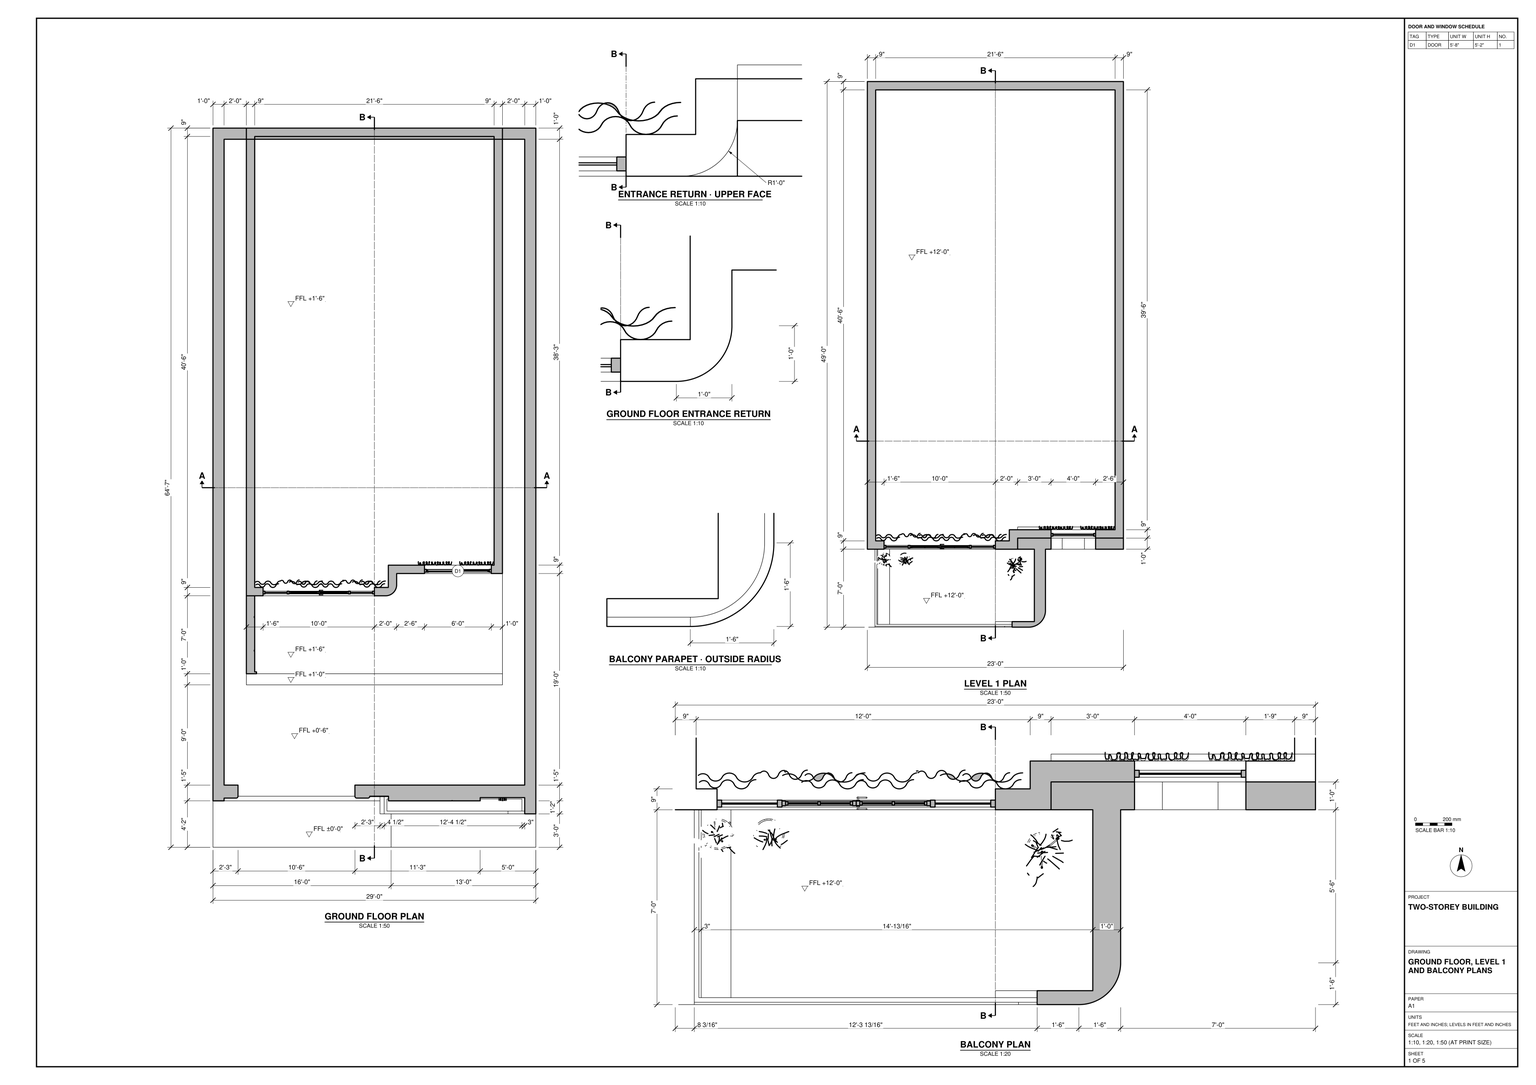
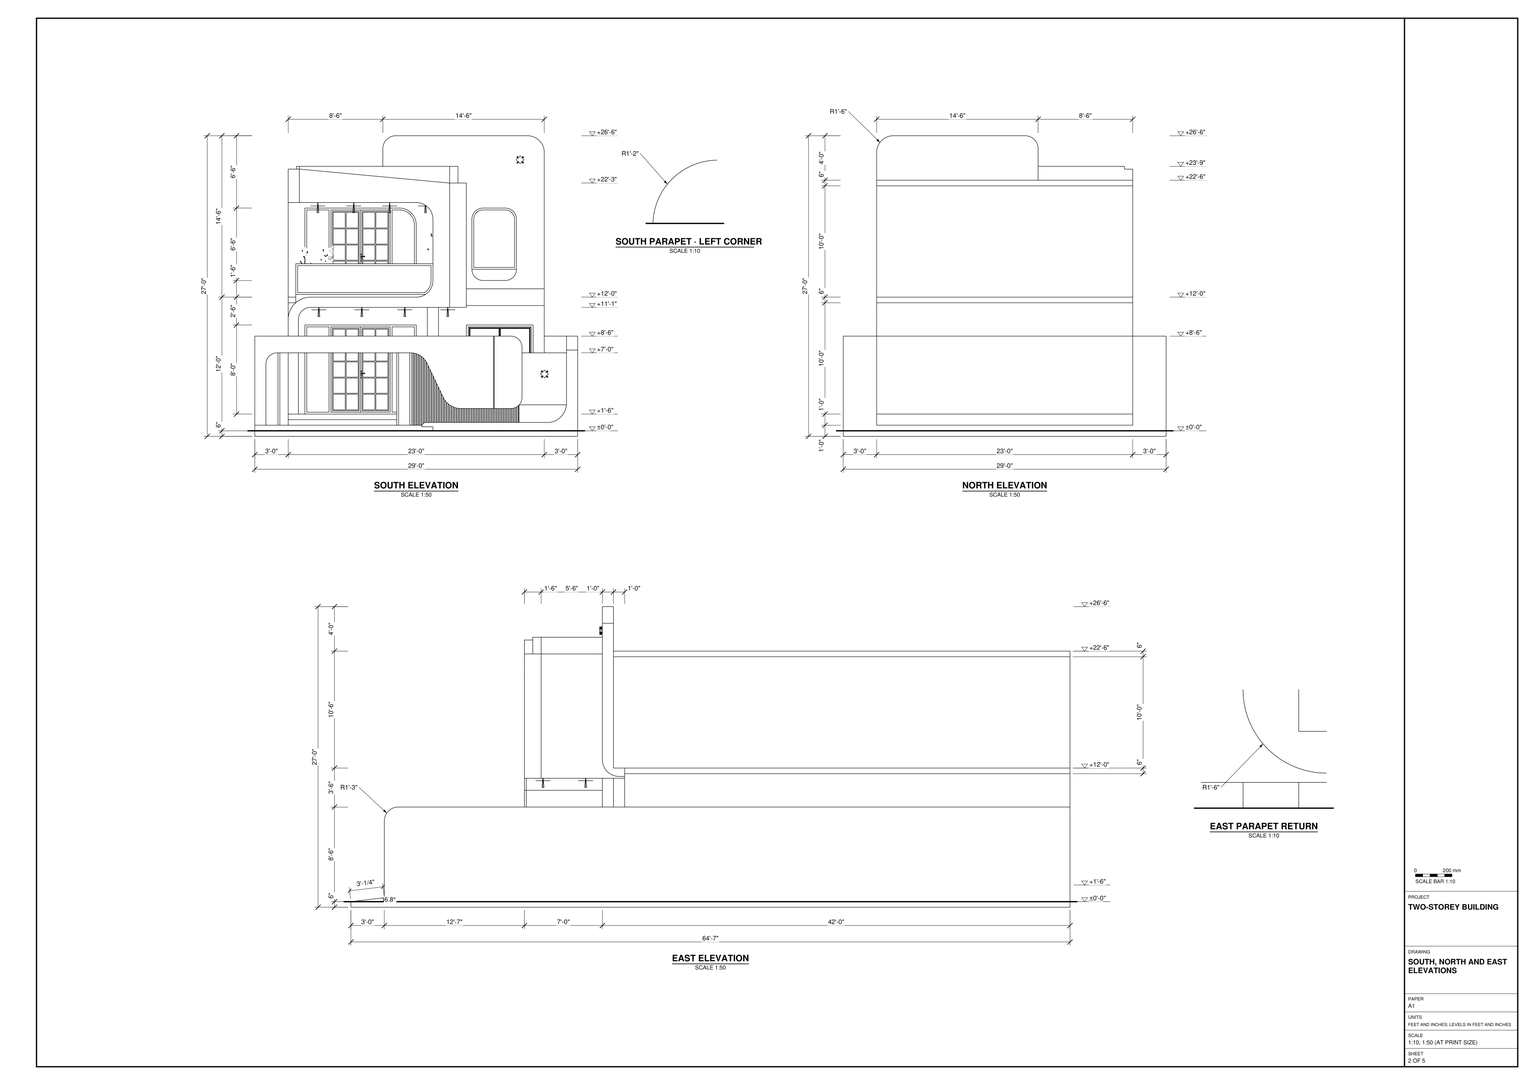
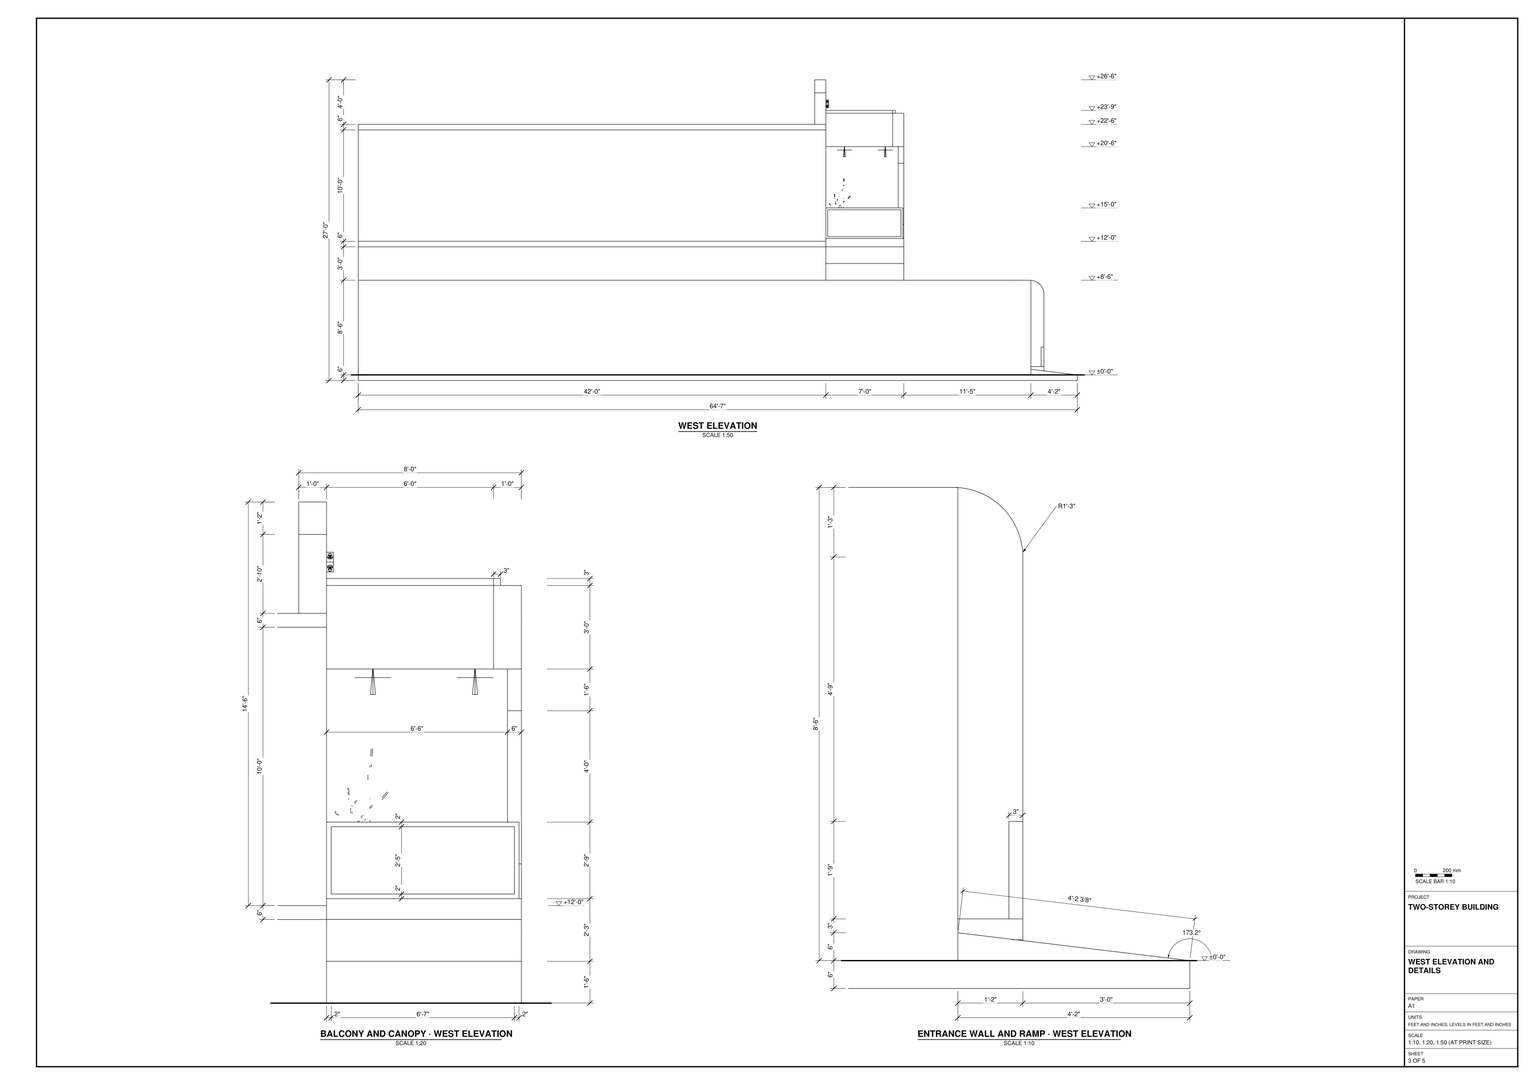
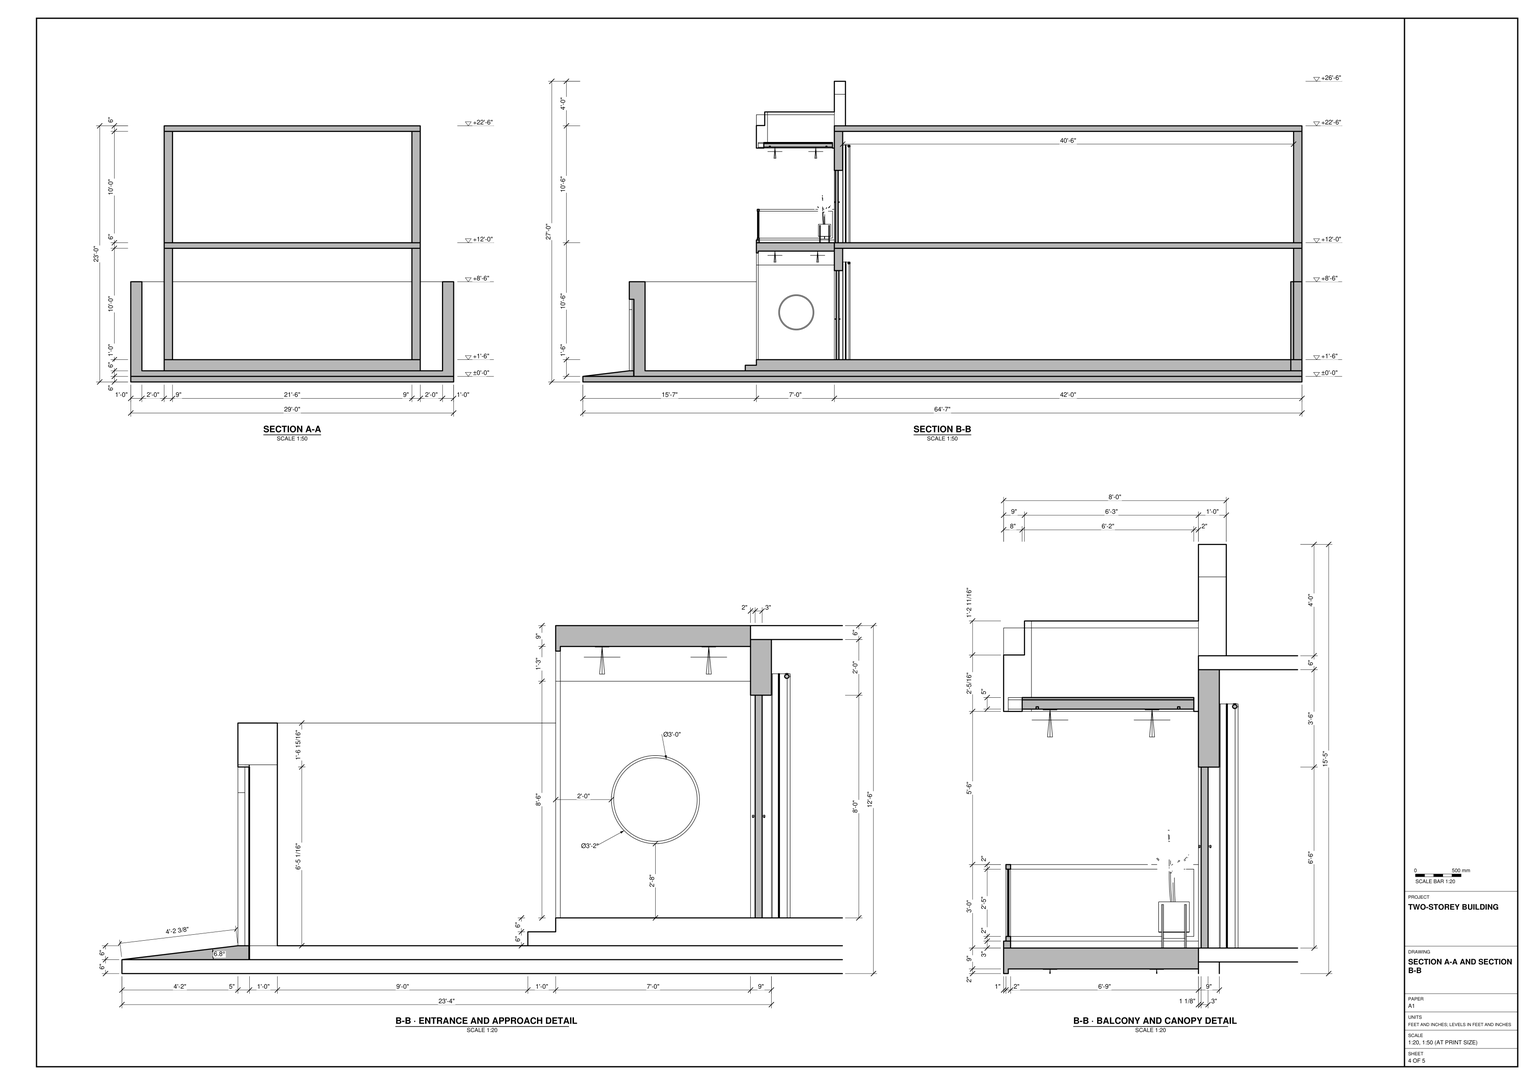
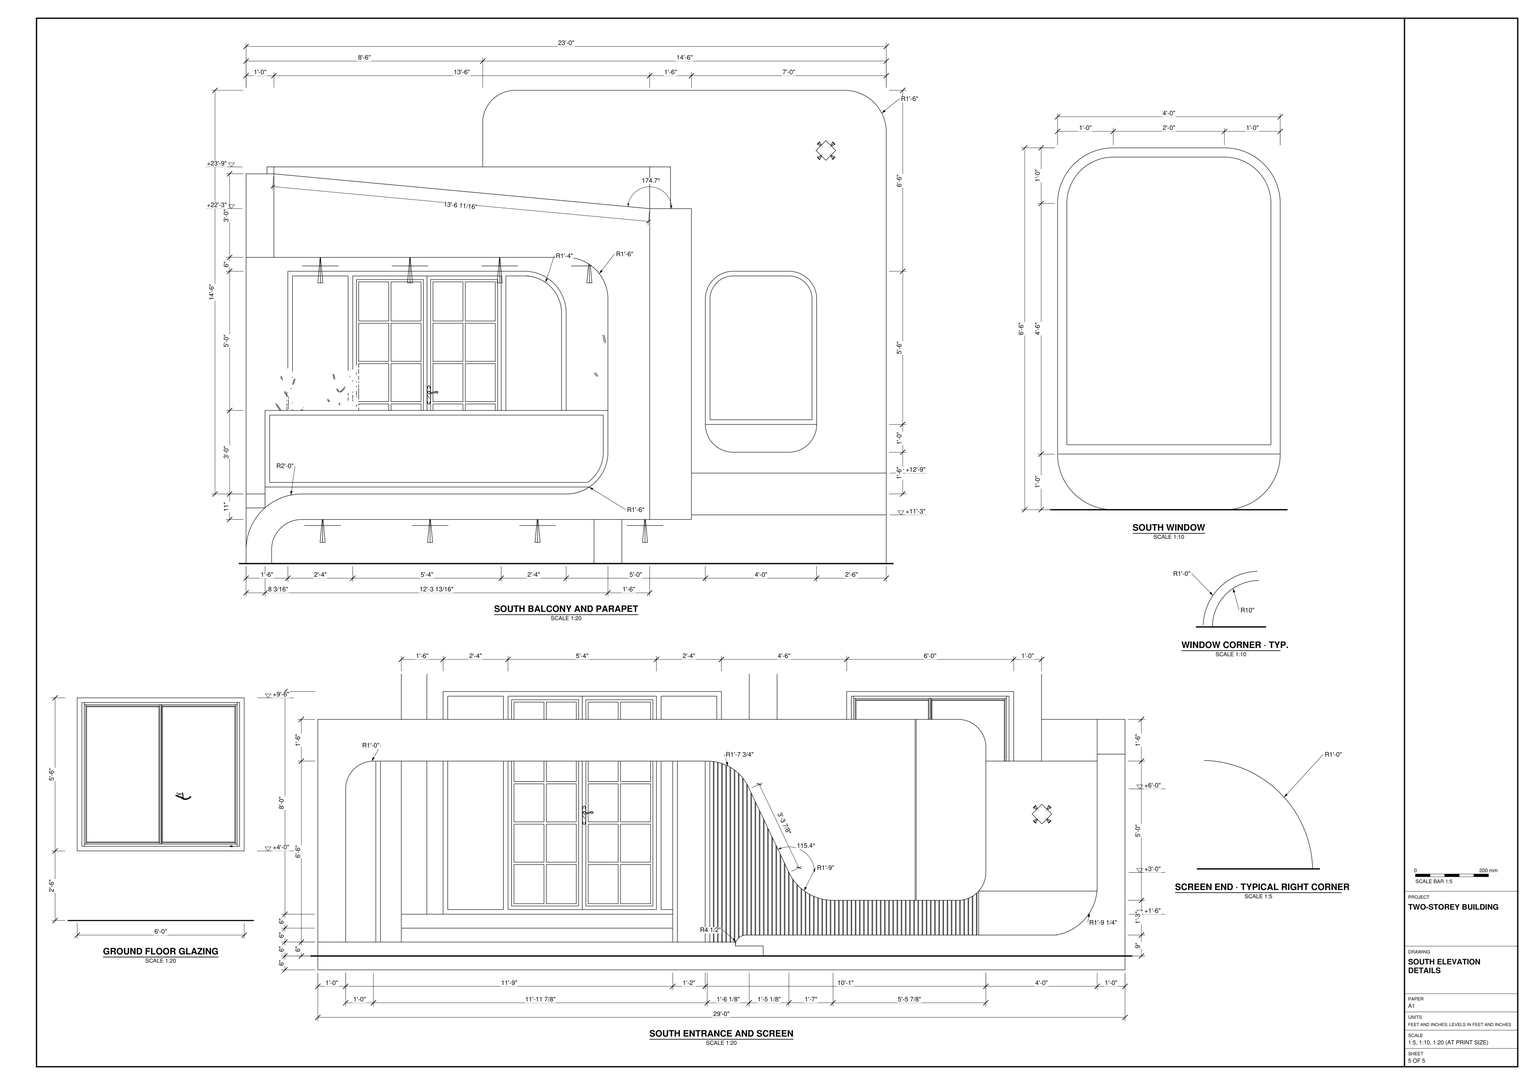
Build the two-storey building in SketchUp from task_files/diagram_01.pdf. Work in feet and inches. Set out the model 29'-0" wide by 64'-7" deep, with an overall height of 27'-0". Use ±0'-0" as the ground datum and +12'-0" for the upper floor. Distinguish the ground datum from the raised entrance floor at +1'-6".

Centre the narrower building shell between the long side boundary walls, leaving the entrance court to the south. Model the walls at their drawn thicknesses, the floor and flat roof slabs, and the stepped front wall line on each storey. Follow the approach from the ramp through the screened court entrance and up the steps to the recessed ground-floor glazing. Fit the door and window units into their openings. Above the entrance, model the projecting balcony, its rounded parapet return and the canopy. Use the south elevation to place the canopy in front of the taller parapet and the separate rounded opening beside the balcony.

Keep walls, slabs and roof in separate groups or components, group each furniture or joinery piece separately where shown, and use components for repeated parts. Decor and loose items, including balcony plants and lights, may be any suitable library components. Save one SketchUp model as output_files/two_storey_building_with_a_front_court_and_balcony.skp.

# SketchUp Ruby script. Lengths in inches.
U = 1.inch
M = Sketchup.active_model
def pt(a) = Geom::Point3d.new(a.map { |v| v * U })
def face(e, loops, mat)
  f = e.add_face(loops[0].map { |a| pt(a) })
  loops[1..].each { |l| e.add_face(l.map { |a| pt(a) }).erase! }
  f.material = f.back_material = mat if mat
  f
end
# faces: each face lists its corners as indices into pts; further lists are holes
def faces(e, pts, list, mat = nil) = list.each { |f| face(e, (f[0].is_a?(Array) ? f : [f]).map { |l| l.map { |i| pts[i] } }, mat) }
# xy, xz, yz: faces in a plane at the given z, y or x. An outline is a flat list of corners, or four numbers for a rectangle; further outlines are holes
def ring(l) = l.size == 4 ? [[l[0], l[1]], [l[2], l[1]], [l[2], l[3]], [l[0], l[3]]] : l.each_slice(2).to_a
def flat(e, list, mat, &to3) = list.each { |f| face(e, (f[0].is_a?(Array) ? f : [f]).map { |l| ring(l).map { |u, v| to3.(u, v) } }, mat) }
def xy(e, z, list, mat = nil) = flat(e, list, mat) { |x, y| [x, y, z] }
def xz(e, y, list, mat = nil) = flat(e, list, mat) { |x, z| [x, y, z] }
def yz(e, x, list, mat = nil) = flat(e, list, mat) { |y, z| [x, y, z] }
def lines(e, pts, list) = list.each { |a, b| e.add_line(pt(pts[a]), pt(pts[b])) }
# prism: a flat outline (further loops are holes) pulled along v
def prism(e, loops, v, mat = nil)
  f = face(e, loops, mat); d = Geom::Vector3d.new(v.map { |x| x * U })
  f.pushpull(f.normal.samedirection?(d) ? d.length : -d.length)
end
def box(e, o, s, mat = nil) = prism(e, [[o, [o[0] + s[0], o[1], o[2]], [o[0] + s[0], o[1] + s[1], o[2]], [o[0], o[1] + s[1], o[2]]]], [0, 0, s[2]], mat)
def at(x, y, z, deg = 0) = Geom::Transformation.translation(pt([x, y, z])) * Geom::Transformation.rotation(ORIGIN, Z_AXIS, deg.degrees)
def axes(o, x, y, z) = Geom::Transformation.new([*x, 0, *y, 0, *z, 0, *pt(o).to_a, 1])
def part(name) = M.definitions.add(name)
# library, detail: a bought-in or finely detailed component or shape, given as its bounding box
def library(name, o, s) = part(name).tap { |d| box(d.entities, o, s) }
def detail(e, o, s) = box(e.add_group.entities, o, s)
def put(e, d, t, mat = nil) = e.add_instance(d, t).tap { |i| i.material = mat if mat }
def group(e, t, mat = nil) = e.add_group.tap { |g| g.transformation = t; g.material = mat if mat }.entities
root = M.entities
M.materials.add("1421 AP 8232 ELEGANT GREY").color = [96, 96, 96]
M.materials.add("BANANA_BIG_STVOL_1").color = [93, 83, 53]
M.materials.add("POT_TEXTURE_1").color = [172, 172, 172]
M.materials.add("POT_TEXTURE_2").color = [160, 154, 144]
M.materials.add("soil1").color = [68, 55, 47]
M.materials.add("white_concrete_pot1").color = [212, 211, 204]
M.materials.add("wood_1").color = [140, 119, 94]
c1 = library("Mixed flower bed",[0,-29.95,0],[46.06,29.95,37.97])
c2 = library("Group\#85",[-312.76,2118.02,370.79],[80.37,61.43,57.53])
c3 = library("Group\#88",[-161.07,2117.49,373.61],[81.25,53.73,39.48])
c4 = library("Group\#89",[-202.35,1900.5,372.29],[58.53,80.11,50.06])
c5 = library("Group\#92",[-148.5,2084.1,354.63],[73.89,71.73,39.48])
c6 = library("Group\#94",[-392.38,2142.99,345.23],[79.77,60.6,39.05])
c7 = library("Group\#95",[-433.57,2042.61,369.7],[71.79,72.8,37.85])
c8 = library("Group\#96",[-374.28,1979.7,369.99],[51.81,82.66,37.9])
c9 = library("Group\#97",[-432.01,1984.38,372.6875],[64.1,75.95,39.0625])
c10 = library("Group\#98",[-389.63,2051.04,359.41],[56.81,81.38,37.86])
c11 = library("Group\#101",[-435.875,2067.96,347.82],[58.32,80.53,38.29])
c12 = library("Group\#102",[-362.86,1963.26,351.01],[55.56,80.44,37.9])
c13 = library("Group\#104",[-330.83,2117.69,370.2],[61.83,80.2,35.55])
c14 = library("Group\#105",[-200.52,1998.86,370.22],[77.15,68.38,35.39])
c15 = library("Group\#106",[-146.29,2044.53,349.125],[81,53.32,37.9])
c16 = library("Group\#109",[-340.96,1970.4,361.28],[81.22,51.59,61.62])
c17 = library("Group\#110",[-310.7,1952.62,354.63],[79.53,58.52,39.48])
c18 = library("Group\#111",[-143.56,2061.14,371.42],[79.79,63.19,51.3])
c19 = library("Group\#113",[-145.08,2015.32,369.99],[82.29,54.05,37.9])
c20 = library("Group\#115",[-272.7,1884.51,369.99],[80.39,55.87,37.9])
c21 = library("Group\#117",[-480.58,1843.32,11.96],[467.85,466.24,378.92])
c22 = library("Group\#120",[-363.89,1895.22,354.63],[76.92,66.54,39.48])
c23 = library("Group\#121",[-390.04,2074.71,363.78],[77.3,84.83,61.55])
c24 = library("Group\#122",[-419.21,1941.11,355.02],[73.1,71.21,39.06])
c25 = library("Group\#125",[-229.79,1894.04,351.01],[79.82,63.55,37.9])
c26 = library("Group\#127",[-397.18,1916.74,372.44],[70.02,74.57,49.25])
c27 = library("Group\#129",[-315.77,2202.04,371],[80.74,54.44,37.85])
c28 = library("Group\#131",[-372.4375,2154.5,374],[76.125,67.08,39.0625])
c29 = library("Group\#132",[-275.5,2156.34,352.11],[71.39,73.27,44.69])
c30 = library("Group\#133",[-183.79,2161.45,371.25],[72.43,70.21,54.35])
c31 = library("Group\#134",[-236.3,2186.8,344.47],[79.26,62.91,39.06])
c32 = library("Group\#135",[-366.3125,2177.8,359.41],[79.9,61.23,37.86])
c33 = library("Group\#136",[-234.26,2180.97,367.05],[50.63,74.65,43.95])
c34 = library("Group\#137",[-431.9,1883.46,368.72],[373.65,376.39,18.61])
c35 = library("Group\#138",[-904.81,1865.01,156.3],[624.43,217.34,1227.7])
c36 = library("Group\#139",[-312.51,1611.52,263.78],[120.52,408.52,1275.1])
c37 = library("Group\#140",[-571.16,1736.08,232.33],[294.08,306.57,1438.75])
c38 = library("Group\#141",[-208.23,2037.18,75.37],[621.09,225.61,1251.82])
c39 = library("Group\#142",[-273.21,1593.22,47.51],[374.54,419.07,1416.6])
c40 = library("Group\#143",[-527.15,2088.47,150.96],[267.01,328.12,1599.25])
c41 = library("Group\#144",[-675.58,1862.05,152.55],[378.81,196.01,1743.84])
c42 = library("Group\#145",[-257.06,2048.08,160.05],[394.6,177.93,1743.83])
c43 = library("Group\#146",[-344.84,1500.61,160.55],[176.35,551.19,1921.45])
c44 = library("Group\#147",[-231.77,1913.24,119.96],[448.93,143.84,1582.05])
c45 = library("Group\#148",[-616.67,2098.6,178.29],[331.19,111.16,1177.92])
c46 = library("Group\#149",[-236.03,2064.57,238.29],[378.97,266.89,1422.96])
c47 = library("Group\#150",[-792.12,2067.32,152.13],[549.56,259.52,1931.8])
c48 = library("Group\#151",[-281.17,2118.67,243.77],[133.23,408.71,1313.3])
c49 = library("Group\#152",[-468.76,669.89,380.1875],[424.36,427.47,41.99])
c50 = library("Group\#153",[-516.34,626.77,-4.5625],[517.73,515.95,418.98])
c51 = library("Group\#154",[-445.29,890.31,329.28],[284.3,304.08,2023.29])
c52 = library("Group\#155",[-277.97,488.68,287.26],[362.84,405.94,1768.54])
c53 = library("Group\#156",[-1038.76,656.55,345.34],[733.18,460.51,2065.7])
c54 = library("Group\#157",[-733.48,439.625,202.64],[456.28,533.12,1536.78])
c55 = library("Group\#158",[-249.24,914.85,310.18],[345.55,647.95,1307.93])
c56 = library("Group\#159",[-662.41,217.3,320.04],[397.32,658.3,1732.06])
c57 = library("Group\#160",[-455.56,899.32,410.78],[341.21,610.33,1581.5])
c58 = library("Group\#161",[-299.2,181.55,262.58],[360.65,735.71,1258.34])
c59 = library("Group\#162",[-258.04,-282.68,604.05],[115.53,137.01,52.63])
c60 = library("Group\#163",[-447.02,-464.95,536.35],[343.73,346.24,39.39])
c61 = library("Group\#164",[-394.9,-448.99,911.74],[90.19,96.88,85.93])
c62 = library("Group\#165",[-246.45,-349.05,558.47],[136.91,100.49,66.1])
c63 = library("Group\#166",[-249.18,-250.59,980.93],[152.21,116.16,134.05])
c64 = library("Group\#167",[-438.92,-265.61,702.3],[171.52,146.16,133.5])
c65 = library("Group\#168",[-264.68,-415.73,1484.11],[304.64,209.69,227.41])
c66 = library("Group\#169",[-545.09,-386.51,922.3125],[300.25,219.65,227.33])
c67 = library("Group\#170",[-304.79,-269.16,622.65],[82.06,111.89,102.57])
c68 = library("Group\#171",[-292.14,-288.9,1281.79],[169.55,204.34,203.36])
c69 = library("Group\#172",[-244.55,-305.59,1009.46],[103.13,76.81,77.34])
c70 = library("Group\#173",[-341.93,-403.49,744.8125],[64.83,96.32,132.15])
c71 = library("Group\#174",[-424,-312.27,817.53],[158.81,108.06,136.45])
c72 = library("Group\#175",[-357.04,-394.18,1447.05],[213.62,306.36,356.95])
c73 = library("Group\#176",[-568.91,-444.37,1285.4],[307.6,179.39,277.93])
c74 = library("Group\#177",[-388.93,-514.39,838.93],[89.79,77.73,82.08])
c75 = library("Group\#178",[-409.02,-515.05,915.53],[69.62,77.27,65.47])
c76 = library("Group\#179",[-295.03,-516.52,742.34],[68.71,141.75,78.67])
c77 = library("Group\#180",[-498.98,-524.4,908.45],[120.83,107.95,112.98])
c78 = library("Group\#181",[-278.4,-571.99,1530.91],[311.57,345.77,423.62])
c79 = library("Group\#182",[-548.25,-262.82,1459.54],[373.26,352.35,568])
c80 = library("Group\#183",[-321.08,-139.66,1308.49],[285.55,393.29,221.53])
c81 = library("Group\#184",[-387.74,-136.11,1470.07],[230,321.58,230.27])
c82 = library("Group\#185",[-293.78,-482.77,597.9],[158.75,112.78,159.87])
c83 = library("Group\#186",[-422.77,-235.4,843.61],[178.54,197.77,233.54])
c84 = library("Group\#187",[-292.81,-667.38,1418.14],[215.17,356.07,188.87])
c85 = library("Group\#188",[-385.21,-446.52,494.02],[160.93,321.12,1142.36])
c86 = library("Group\#189",[-492.14,-508.4,-4.15],[433.72,431.71,567.03])
c87 = library("Group\#190",[-429.18,-1441.17,362.05],[345.84,348.28,45.35])
c88 = library("Group\#191",[-487.23,-1483.58,-4.71],[450.86,446.99,418.38])
c89 = library("Group\#192",[-513.94,-1201.2,195.17],[480.66,557.42,1160.08])
c90 = library("Group\#193",[-545.36,-1775.03,287.125],[412.21,432,920.68])
c91 = library("Group\#194",[-208.03,-1336.63,286.21],[381.72,484.79,1145.39])
c92 = library("Group\#195",[-163.65,-1622.09,292.29],[406.18,374.8,780.12])
c93 = library("Group\#196",[-245.33,-1174.2,301.22],[356.02,306.31,608.34])
c94 = library("Group\#197",[-640.625,-1318.37,287.11],[396.64,314.81,689.96])
c95 = library("Group\#198",[-750.24,-1478.51,301.56],[423.84,451.05,998.69])
c96 = library("Group\#199",[-426.76,-1753.59,287.48],[479.67,412.35,1049.19])
c97 = library("Group\#200",[-619.83,-1636.3,288.9],[316.15,456.61,1171.28])
c98 = library("Group\#201",[-738.91,-1210.08,301],[426.4,388.88,1000.79])
c99 = library("Group\#202",[-172.82,-1329.68,294.68],[502.85,397.72,955.79])
c100 = library("Group\#203",[-208.33,-1511.76,297.04],[508.2,421.96,1258.76])
c101 = library("Group\#204",[-384.8,-1640.99,300.61],[422.68,348.03,1297.96])
c102 = library("Group\#205",[-445.7,-1606.55,154.18],[255.44,283.57,849.28])
c103 = library("Group\#206",[-390.1,-1177.12,195.59],[220.93,265.44,790.12])
c104 = library("Group\#207",[-208.0625,-1498.77,286.27],[547.26,435.76,1075.6])
c105 = library("Group\#208",[-480.32,-1333.42,295.8],[424.49,356.06,1482.77])
c106 = library("Group\#209",[-378.01,-1245.98,305.66],[422.15,474.55,1267.42])
c107 = library("Group\#210",[-480.3,-2300.47,677.45],[398.14,398.43,28.25])
c108 = library("Group\#211",[-336.38,-2175.79,614.41],[133.99,147.1,560.64])
c109 = library("Group\#212",[-311.45,-2362.85,663.67],[597.01,322.07,1007.38])
c110 = library("Group\#213",[-330.26,-2159.14,612.04],[116.66,119.22,673.97])
c111 = library("Group\#214",[-667.53,-2111.4375,1071.74],[420.02,555.28,968.03])
c112 = library("Group\#215",[-328.97,-2115.58,1156.29],[117.86,119.42,695.38])
c113 = library("Group\#216",[-943.22,-2312.1875,967.59],[670.63,402.45,1245.73])
c114 = library("Group\#217",[-568.09,-2386.9,-3.76],[573.62,569.18,700.28])
c115 = library("Group\#218",[-343.93,-2076.42,1024.91],[285.05,475.82,708.21])
c116 = library("Group\#219",[-550.09,-2664.39,1031.96],[371.42,533.86,798])
c117 = library("Group\#220",[-308.37,-2556.11,869.35],[483.58,483.6,1385.8])
c118 = part("3d model (27)")
p = [[0,0,0],[1,0,0],[1,1,0]]
lines(c118.entities,p,[[0,1],[1,2],[2,0]])
g1 = group(c118.entities,at(0,0,0),"white_concrete_pot1")
detail(g1,[-222.14,2117.95,372.07],[61.87,75.41,50.35])
g2 = group(c118.entities,at(0,0,0),"white_concrete_pot1")
detail(g2,[-313.93,1881.02,351.21],[70.15,73.18,37.2])
put(c118.entities,c2,at(0,0,0),"white_concrete_pot1")
g3 = group(c118.entities,at(0,0,0),"white_concrete_pot1")
detail(g3,[-214.75,1956.59,330.04],[66.78,77.69,39.48])
g4 = group(c118.entities,at(0,0,0),"white_concrete_pot1")
detail(g4,[-249.82,2117.53,359.91],[58.07,81.25,37.2])
put(c118.entities,c3,at(0,0,0),"white_concrete_pot1")
put(c118.entities,c4,at(0,0,0),"white_concrete_pot1")
g5 = group(c118.entities,at(0,0,0),"white_concrete_pot1")
detail(g5,[-173.8,2126.25,354.63],[80.17,60.53,39.48])
g6 = group(c118.entities,at(0,0,0),"white_concrete_pot1")
detail(g6,[-222.96,2066.75,359.91],[63.77,78.21,37.2])
put(c118.entities,c5,at(0,0,0),"white_concrete_pot1")
g7 = group(c118.entities,at(0,0,0),"white_concrete_pot1")
detail(g7,[-319.36,2078.81,339.18],[76.07,69.08,39.48])
put(c118.entities,c6,at(0,0,0),"white_concrete_pot1")
put(c118.entities,c7,at(0,0,0),"white_concrete_pot1")
put(c118.entities,c8,at(0,0,0),"white_concrete_pot1")
put(c118.entities,c9,at(0,0,0),"white_concrete_pot1")
put(c118.entities,c10,at(0,0,0),"white_concrete_pot1")
g8 = group(c118.entities,at(0,0,0),"white_concrete_pot1")
detail(g8,[-129.49,1972.75,359.91],[55.59,80.76,37.2])
g9 = group(c118.entities,at(0,0,0),"white_concrete_pot1")
detail(g9,[-183.125,1913.38,330.04],[66.78,77.69,39.48])
put(c118.entities,c11,at(0,0,0),"white_concrete_pot1")
put(c118.entities,c12,at(0,0,0),"white_concrete_pot1")
g10 = group(c118.entities,at(0,0,0),"white_concrete_pot1")
detail(g10,[-435.4375,2027.54,350.71],[78.74,62.6,37.86])
put(c118.entities,c13,at(0,0,0),"white_concrete_pot1")
put(c118.entities,c14,at(0,0,0),"white_concrete_pot1")
put(c118.entities,c15,at(0,0,0),"white_concrete_pot1")
g11 = group(c118.entities,at(0,0,0),"white_concrete_pot1")
detail(g11,[-394.5,2036.48,359.91],[79.58,64.84,37.2])
g12 = group(c118.entities,at(0,0,0),"white_concrete_pot1")
detail(g12,[-333.13,1892.25,370.19],[61.39,79.4,37.2])
put(c118.entities,c16,at(0,0,0),"white_concrete_pot1")
put(c118.entities,c17,at(0,0,0),"white_concrete_pot1")
put(c118.entities,c18,at(0,0,0),"white_concrete_pot1")
g13 = group(c118.entities,at(0,0,0),"white_concrete_pot1")
detail(g13,[-195.71,2019.1875,371.11],[58.98,81.18,37.2])
put(c118.entities,c19,at(0,0,0),"white_concrete_pot1")
g14 = group(c118.entities,at(0,0,0),"white_concrete_pot1")
detail(g14,[-282.5625,1934.21,389.56],[81.1,59.19,35.03])
put(c118.entities,c20,at(0,0,0),"white_concrete_pot1")
g15 = group(c118.entities,at(0,0,0),"white_concrete_pot1")
detail(g15,[-240.6,2054.85,378.89],[71.5,72.03,37.2])
put(c118.entities,c21,at(0,0,0),"POT_TEXTURE_1")
g16 = group(c118.entities,at(0,0,0),"white_concrete_pot1")
detail(g16,[-209.1,1970.26,378.89],[50.57,81.04,37.2])
g17 = group(c118.entities,at(0,0,0),"white_concrete_pot1")
detail(g17,[-417.64,2112.53,369.82],[65.44,79.59,38.29])
put(c118.entities,c22,at(0,0,0),"white_concrete_pot1")
put(c118.entities,c23,at(0,0,0),"white_concrete_pot1")
put(c118.entities,c24,at(0,0,0),"white_concrete_pot1")
g18 = group(c118.entities,at(0,0,0),"white_concrete_pot1")
detail(g18,[-152,1936.85,378.89],[64.46,79.76,37.2])
g19 = group(c118.entities,at(0,0,0),"white_concrete_pot1")
detail(g19,[-284.65,1933.22,373.64],[80.83,55.23,37.2])
put(c118.entities,c25,at(0,0,0),"white_concrete_pot1")
g20 = group(c118.entities,at(0,0,0),"white_concrete_pot1")
detail(g20,[-263.49,1923.54,359.91],[75.98,66.75,37.2])
put(c118.entities,c26,at(0,0,0),"white_concrete_pot1")
g21 = group(c118.entities,at(0,0,0),"white_concrete_pot1")
detail(g21,[-167.97,1940.97,354.63],[66.78,77.7,39.48])
put(c118.entities,c27,at(0,0,0),"white_concrete_pot1")
g22 = group(c118.entities,at(0,0,0),"white_concrete_pot1")
detail(g22,[-270.91,2176.57,345.18],[52.11,82.01,38.29])
put(c118.entities,c28,at(0,0,0),"white_concrete_pot1")
put(c118.entities,c29,at(0,0,0),"white_concrete_pot1")
put(c118.entities,c30,at(0,0,0),"white_concrete_pot1")
put(c118.entities,c31,at(0,0,0),"white_concrete_pot1")
put(c118.entities,c32,at(0,0,0),"white_concrete_pot1")
put(c118.entities,c33,at(0,0,0),"white_concrete_pot1")
put(c118.entities,c34,at(0,0,0),"white_concrete_pot1")
put(c118.entities,c35,at(0,0,0))
put(c118.entities,c36,at(0,0,0))
put(c118.entities,c37,at(0,0,0))
put(c118.entities,c38,at(0,0,0))
put(c118.entities,c39,at(0,0,0))
put(c118.entities,c40,at(0,0,0))
put(c118.entities,c41,at(0,0,0))
put(c118.entities,c42,at(0,0,0))
put(c118.entities,c43,at(0,0,0))
put(c118.entities,c44,at(0,0,0))
put(c118.entities,c45,at(0,0,0))
put(c118.entities,c46,at(0,0,0))
put(c118.entities,c47,at(0,0,0))
put(c118.entities,c48,at(0,0,0))
put(c118.entities,c49,at(0,0,0),"soil1")
put(c118.entities,c50,at(0,0,0),"POT_TEXTURE_1")
put(c118.entities,c51,at(0,0,0))
put(c118.entities,c52,at(0,0,0))
put(c118.entities,c53,at(0,0,0))
put(c118.entities,c54,at(0,0,0))
put(c118.entities,c55,at(0,0,0))
put(c118.entities,c56,at(0,0,0))
put(c118.entities,c57,at(0,0,0))
put(c118.entities,c58,at(0,0,0))
put(c118.entities,c59,at(0,0,0))
put(c118.entities,c60,at(0,0,0),"soil1")
put(c118.entities,c61,at(0,0,0))
put(c118.entities,c62,at(0,0,0))
put(c118.entities,c63,at(0,0,0))
put(c118.entities,c64,at(0,0,0))
put(c118.entities,c65,at(0,0,0))
put(c118.entities,c66,at(0,0,0))
put(c118.entities,c67,at(0,0,0))
put(c118.entities,c68,at(0,0,0))
put(c118.entities,c69,at(0,0,0))
put(c118.entities,c70,at(0,0,0))
put(c118.entities,c71,at(0,0,0))
put(c118.entities,c72,at(0,0,0))
put(c118.entities,c73,at(0,0,0))
put(c118.entities,c74,at(0,0,0))
put(c118.entities,c75,at(0,0,0))
put(c118.entities,c76,at(0,0,0))
put(c118.entities,c77,at(0,0,0))
put(c118.entities,c78,at(0,0,0))
put(c118.entities,c79,at(0,0,0))
put(c118.entities,c80,at(0,0,0))
put(c118.entities,c81,at(0,0,0))
put(c118.entities,c82,at(0,0,0))
put(c118.entities,c83,at(0,0,0))
put(c118.entities,c84,at(0,0,0))
put(c118.entities,c85,at(0,0,0),"wood_1")
put(c118.entities,c86,at(0,0,0),"POT_TEXTURE_2")
put(c118.entities,c87,at(0,0,0),"soil1")
put(c118.entities,c88,at(0,0,0),"POT_TEXTURE_1")
put(c118.entities,c89,at(0,0,0))
put(c118.entities,c90,at(0,0,0))
put(c118.entities,c91,at(0,0,0))
put(c118.entities,c92,at(0,0,0))
put(c118.entities,c93,at(0,0,0))
put(c118.entities,c94,at(0,0,0))
put(c118.entities,c95,at(0,0,0))
put(c118.entities,c96,at(0,0,0))
put(c118.entities,c97,at(0,0,0))
put(c118.entities,c98,at(0,0,0))
put(c118.entities,c99,at(0,0,0))
put(c118.entities,c100,at(0,0,0))
put(c118.entities,c101,at(0,0,0))
put(c118.entities,c102,at(0,0,0))
put(c118.entities,c103,at(0,0,0))
put(c118.entities,c104,at(0,0,0))
put(c118.entities,c105,at(0,0,0))
put(c118.entities,c106,at(0,0,0))
put(c118.entities,c107,at(0,0,0),"soil1")
put(c118.entities,c108,at(0,0,0),"BANANA_BIG_STVOL_1")
put(c118.entities,c109,at(0,0,0))
put(c118.entities,c110,at(0,0,0),"BANANA_BIG_STVOL_1")
put(c118.entities,c111,at(0,0,0))
put(c118.entities,c112,at(0,0,0))
put(c118.entities,c113,at(0,0,0))
put(c118.entities,c114,at(0,0,0),"POT_TEXTURE_2")
put(c118.entities,c115,at(0,0,0))
put(c118.entities,c116,at(0,0,0))
put(c118.entities,c117,at(0,0,0))
c119 = library("Group\#7",[-4.36,-62.89,0],[280.36,542.89,120])
c120 = library("Group\#11",[0,0,0],[276,504,6])
c121 = library("Group\#2",[0,-24,0],[276,504,120])
c122 = library("Group\#15",[-36,-175,-6],[348,775,102])
c123 = library("Group\#13",[0,0,0],[276,108,300])
g23 = group(root,at(36,295,0))
put(g23,c1,axes([254.43,-243,-17],[1,0,0],[0,0.43409,0],[0,0,1]))
g24 = group(g23,at(-36,-240,-18))
put(g24,c118,axes([253.68,218.14,18.11],[0,-0.02318,0],[0.02157,0,0],[0,0,0.02333]))
put(g24,c119,at(36,240,144))
g25 = group(g24,at(36,216,18))
prism(g25,[[[0,-84,0],[0,504,0],[0,504,-12],[0,-96,-12],[0,-96,-6],[0,-84,-6]]],[276,0,0])
put(g24,c120,at(36,216,138))
g26 = group(g24,at(36,216,264))
prism(g26,[[[276,504,0],[276,12,0],[162,12,0],[162,0,0],[0,0,0],[0,504,0]]],[0,0,6])
put(g24,c121,at(36,240,18),"1421 AP 8232 ELEGANT GREY")
put(g24,c122,at(36,120,6))
put(g24,c123,at(36,132,18))
g27 = group(g24,at(0,-55,0))
box(g27,[0,0,-6],[348,775,6])
